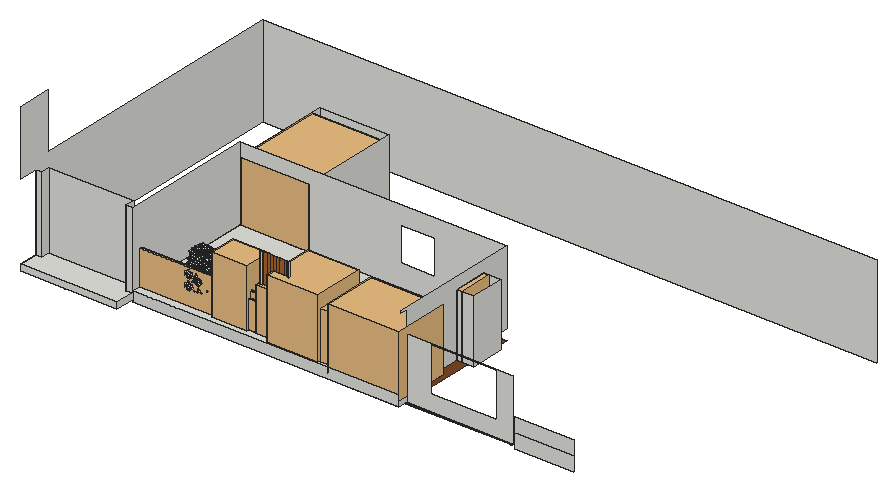
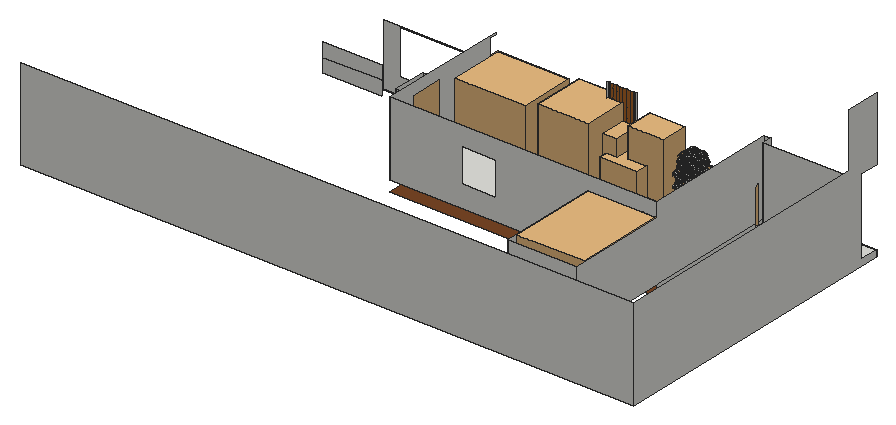
# SketchUp Ruby script. Lengths in inches.
U = 1.inch
M = Sketchup.active_model
def pt(a) = Geom::Point3d.new(a.map { |v| v * U })
def face(e, loops, mat)
  f = e.add_face(loops[0].map { |a| pt(a) })
  loops[1..].each { |l| e.add_face(l.map { |a| pt(a) }).erase! }
  f.material = f.back_material = mat if mat
  f
end
# faces: each face lists its corners as indices into pts; further lists are holes
def faces(e, pts, list, mat = nil) = list.each { |f| face(e, (f[0].is_a?(Array) ? f : [f]).map { |l| l.map { |i| pts[i] } }, mat) }
# xy, xz, yz: faces in a plane at the given z, y or x. An outline is a flat list of corners, or four numbers for a rectangle; further outlines are holes
def ring(l) = l.size == 4 ? [[l[0], l[1]], [l[2], l[1]], [l[2], l[3]], [l[0], l[3]]] : l.each_slice(2).to_a
def flat(e, list, mat, &to3) = list.each { |f| face(e, (f[0].is_a?(Array) ? f : [f]).map { |l| ring(l).map { |u, v| to3.(u, v) } }, mat) }
def xy(e, z, list, mat = nil) = flat(e, list, mat) { |x, y| [x, y, z] }
def xz(e, y, list, mat = nil) = flat(e, list, mat) { |x, z| [x, y, z] }
def yz(e, x, list, mat = nil) = flat(e, list, mat) { |y, z| [x, y, z] }
def lines(e, pts, list) = list.each { |a, b| e.add_line(pt(pts[a]), pt(pts[b])) }
# prism: a flat outline (further loops are holes) pulled along v
def prism(e, loops, v, mat = nil)
  f = face(e, loops, mat); d = Geom::Vector3d.new(v.map { |x| x * U })
  f.pushpull(f.normal.samedirection?(d) ? d.length : -d.length)
end
def box(e, o, s, mat = nil) = prism(e, [[o, [o[0] + s[0], o[1], o[2]], [o[0] + s[0], o[1] + s[1], o[2]], [o[0], o[1] + s[1], o[2]]]], [0, 0, s[2]], mat)
def at(x, y, z, deg = 0) = Geom::Transformation.translation(pt([x, y, z])) * Geom::Transformation.rotation(ORIGIN, Z_AXIS, deg.degrees)
def axes(o, x, y, z) = Geom::Transformation.new([*x, 0, *y, 0, *z, 0, *pt(o).to_a, 1])
def part(name) = M.definitions.add(name)
# library, detail: a bought-in or finely detailed component or shape, given as its bounding box
def library(name, o, s) = part(name).tap { |d| box(d.entities, o, s) }
def detail(e, o, s) = box(e.add_group.entities, o, s)
def put(e, d, t, mat = nil) = e.add_instance(d, t).tap { |i| i.material = mat if mat }
def group(e, t, mat = nil) = e.add_group.tap { |g| g.transformation = t; g.material = mat if mat }.entities
root = M.entities
M.materials.add("[Wood Bamboo]").color = [173, 103, 41]
M.materials.add("[Wood Veneer 01]").color = [120, 70, 37]
c1 = library("Tlon Light 1950 Ceiling 152 010",[-38.39,-38.39,-3.78],[76.78,76.78,3.41])
c2 = library("Rectangular Planter with Plant",[-49.93,-33.04,0],[93.24,71.01,81.08])
c3 = library("Glass Railings(black Handrails)",[-57.04,-132.55,0],[169.29,2.52,28.17])
c4 = library("Group\#14",[0,0,0],[39.5,117.4375,51.17])
c5 = library("Untitled (14)",[0,0,0],[7.13,36,83])
c6 = library("Hanging Plant\#2",[-3.24,-1.74,-0.87],[34.15,22.4,50.98])
c7 = library("Yukka Plant GHD",[0,0,0],[46.13,35.26,75.51])
c8 = library("Philodendron Plant GHD",[-18.43,-10.97,-1.09],[51.75,39.48,62.43])
c9 = library("Plant Banana",[3.49,5.74,0],[38.27,39.55,56.51])
c10 = library("Potted indoor plant",[-35.72,-28.42,0],[66.31,67.39,78.4375])
c11 = part("leaflet")
p = [[2.87,10.24,0.32],[0.33,13.79,0],[-2.24,10.39,0.32],[-2.2,6.92,0.33],[0.45,0.11,0.33],[2.91,6.86,0.33]]
faces(c11.entities,p,[[0,1,2],[0,2,3,4,5]])
c12 = part("leaf group")
put(c12.entities,c11,axes([4.25,4.04,0.04],[0.8,0,0],[0,0.8,0],[0,0,0.8]))
put(c12.entities,c11,axes([4.5,3.78,0.04],[0.4,0.69282,-0.00011],[-0.69282,0.4,-0.00008],[-0.00001,0.00014,0.8]))
put(c12.entities,c11,axes([4.92,3.9375,0.04],[-0.56569,0.56569,-0.00025],[-0.56569,-0.56569,0.00001],[-0.00017,0.00019,0.8]))
put(c12.entities,c11,axes([4.87,4.38,0.04],[-0.69282,-0.4,-0.0002],[0.4,-0.69282,0.00017],[-0.00026,0.00005,0.8]))
put(c12.entities,c11,axes([4.42,4.45,0.04],[0.20706,-0.77274,-0.00003],[0.77274,0.20706,0.00016],[-0.00015,-0.00007,0.8]))
c13 = part("branch with leaves\#1")
put(c13.entities,c12,axes([2.86,31.23,35.15],[-0.02765,-0.79009,-0.61237],[0.48114,-0.54749,0.68465],[-0.8762,-0.27571,0.39528]))
put(c13.entities,c12,axes([12.72,29.5,24.05],[-0.41566,0.90952,0],[-0.44736,-0.20444,-0.87067],[-0.7919,-0.3619,0.49186]))
put(c13.entities,c12,axes([15.91,15.09,15.29],[-0.51919,0.82474,-0.22414],[0.78767,0.35997,-0.5],[-0.33169,-0.43615,-0.83652]))
put(c13.entities,c12,axes([23.4,16.37,17.31],[0.5,0.75,-0.43301],[0,0.5,0.86603],[0.86603,-0.43301,0.25]))
put(c13.entities,c12,axes([11.3125,8.27,23.62],[1.15,0,0],[0,0.575,0.99593],[0,-0.86603,0.5]))
c14 = part("leaflet\#1")
p = [[0.33,13.79,0],[2.87,10.24,0.32],[-2.24,10.39,0.32],[2.91,6.86,0.33],[0.45,0.11,0.33],[-2.2,6.92,0.33]]
faces(c14.entities,p,[[0,1,2],[2,1,3,4,5]])
c15 = part("leaf group\#1")
put(c15.entities,c14,axes([1.8,0.82,0.04],[-0.56569,0.56569,-0.00025],[-0.33941,-0.33941,0.00001],[-0.00017,0.00019,0.8]))
c16 = part("flower")
put(c16.entities,c15,axes([3.87,3.58,0.87],[0.08758,0.98061,-0.17532],[0.93721,-0.14075,-0.31909],[-0.33758,-0.13637,-0.93137]))
put(c16.entities,c15,axes([3.58,5.87,0.87],[0.98061,-0.08758,-0.17532],[-0.14075,-0.93721,-0.31909],[-0.13637,0.33758,-0.93137]))
put(c16.entities,c15,axes([5.87,6.16,0.87],[-0.08758,-0.98061,-0.17532],[-0.93721,0.14075,-0.31909],[0.33758,0.13637,-0.93137]))
put(c16.entities,c15,axes([6.16,3.87,0.87],[-0.98061,0.08758,-0.17532],[0.14075,0.93721,-0.31909],[0.13637,-0.33758,-0.93137]))
put(c16.entities,c15,axes([4.97,4.02,1.64],[-0.54077,0.62855,-0.55902],[0.78035,0.12673,-0.61237],[-0.31406,-0.76738,-0.55902]))
put(c16.entities,c15,axes([4.08,5.2,1.64],[0.81472,0.15405,-0.55902],[-0.28042,-0.73917,-0.61237],[-0.50754,0.65567,-0.55902]))
put(c16.entities,c15,axes([5.55,5.38,1.64],[-0.27395,-0.78259,-0.55902],[-0.49993,0.61243,-0.61237],[0.8216,0.11171,-0.55902]))
c17 = part("branch")
p = [[0.27,0.14,21.6],[1.15,1.36,21.6],[2.31,4.21,0],[0.54,1.79,0],[1.05,2.55,32.4],[1.34,2.95,32.4]]
faces(c17.entities,p,[[0,1,2,3],[4,5,1,0]])
c18 = part("branch with leaves")
put(c18.entities,c12,axes([29.28,4.46,29.75],[0.70711,0.61237,-0.35355],[-0.27393,0.69819,0.66144],[0.65189,-0.37086,0.66144]))
put(c18.entities,c12,axes([2.86,31.23,35.15],[-0.02765,-0.79009,-0.61237],[0.48114,-0.54749,0.68465],[-0.8762,-0.27571,0.39528]))
put(c18.entities,c17,axes([15.22,43.9,5.2],[1,0,0],[0,0.5,0.86603],[0,-1.03923,0.6]))
put(c18.entities,c12,axes([12.72,29.5,24.05],[-0.41566,0.90952,0],[-0.44736,-0.20444,-0.87067],[-0.7919,-0.3619,0.49186]))
put(c18.entities,c12,axes([15.91,15.09,15.29],[-0.51919,0.82474,-0.22414],[0.78767,0.35997,-0.5],[-0.33169,-0.43615,-0.83652]))
put(c18.entities,c12,axes([31.61,42.03,14.23],[-0.02765,-0.79009,-0.61237],[0.47126,0.52995,-0.70503],[0.88156,-0.30808,0.35768]))
put(c18.entities,c12,axes([23.4,16.37,17.31],[0.5,0.75,-0.43301],[0,0.5,0.86603],[0.86603,-0.43301,0.25]))
put(c18.entities,c12,axes([12.04,8.6,24.1875],[1,0,0],[0,0.5,0.86603],[0,-0.86603,0.5]))
c19 = part("trunk")
p = [[2.07,0,0],[2.91,2.57,208.4],[2.76,2.68,208.4],[0.57,1.09,0],[3.93,0,0],[3.09,2.57,208.4],
  [5.43,1.09,0],[3.24,2.68,208.4],[2.7,2.85,208.4],[0,2.85,0],[6,2.85,0],[3.3,2.85,208.4],
  [2.76,3.03,208.4],[0.57,4.62,0],[5.43,4.62,0],[3.24,3.03,208.4],[2.91,3.14,208.4],[2.07,5.71,0],
  [3.93,5.71,0],[3.09,3.14,208.4]]
faces(c19.entities,p,[[0,1,2,3],[4,5,1,0],[6,7,5,4],[3,2,8,9],[6,10,11,7],[8,12,13,9],[11,10,14,15],[13,12,16,17],
  [18,19,15,14],[17,16,19,18]])
c20 = part("Flowering tree")
put(c20.entities,c13,axes([8.5625,69.79,58.85],[-1.14545,-0.10223,0],[0.09875,-1.10642,-0.25882],[0.02646,-0.29646,0.96593]))
put(c20.entities,c16,axes([18.03,-59.9,126.47],[-1.06473,0.02061,0.37747],[-0.32263,-0.80708,-0.6548],[0.29115,-0.81896,0.6548]))
put(c20.entities,c16,axes([24.99,-51.52,163.52],[0.99593,0.2875,-0.43301],[0,0.99593,0.5],[0.575,-0.49796,0.75]))
put(c20.entities,c16,axes([9.15,43.86,180.9375],[-0.776,0.32151,0.68301],[0.59221,-0.55726,0.70711],[0.60796,0.9532,0.18301]))
put(c20.entities,c16,axes([-19.44,51.82,88.4375],[-0.978,0.2192,-0.49033],[-0.25151,-1.12216,0],[-0.55023,0.12332,0.87153]))
put(c20.entities,c13,axes([79.24,-48.01,132.64],[0.21275,1.12031,-0.12941],[-1.10684,0.17595,-0.22414],[-0.22834,0.19092,0.96593]))
put(c20.entities,c13,axes([64.36,-6.43,165.85],[-0.10223,1.14545,0],[-1.10642,-0.09875,-0.25882],[-0.29646,-0.02646,0.96593]))
put(c20.entities,c13,axes([52.57,39.62,163.85],[-0.88224,0.73767,0],[-0.71253,-0.85218,-0.25882],[-0.19092,-0.22834,0.96593]))
put(c20.entities,c13,axes([-64.4,-29.26,175.85],[0.88224,-0.73767,0],[0.71253,0.85218,-0.25882],[0.19092,0.22834,0.96593]))
put(c20.entities,c13,axes([40.35,-16.55,200.81],[-0.14358,1.14093,0.01256],[-0.77283,-0.08933,-0.72016],[-0.83795,-0.11311,0.69546]))
put(c20.entities,c13,axes([7.875,84.56,112.85],[-1.14773,-0.07221,0],[0.06975,-1.10862,-0.25882],[0.01869,-0.29705,0.96593]))
put(c20.entities,c13,axes([-66.42,6.43,163.85],[0.10223,-1.14545,0],[1.10642,0.09875,-0.25882],[0.29646,0.02646,0.96593]))
put(c20.entities,c13,axes([-6.02,-66.82,162.85],[1.14545,0.10223,0],[-0.09875,1.10642,-0.25882],[-0.02646,0.29646,0.96593]))
put(c20.entities,c13,axes([65.22,55.72,70.85],[-0.88224,0.73767,0],[-0.71253,-0.85218,-0.25882],[-0.19092,-0.22834,0.96593]))
put(c20.entities,c13,axes([-6.02,-85.22,100.85],[1.14545,0.10223,0],[-0.09875,1.10642,-0.25882],[-0.02646,0.29646,0.96593]))
put(c20.entities,c13,axes([-64.4,-55.71,70.85],[0.88224,-0.73767,0],[0.71253,0.85218,-0.25882],[0.19092,0.22834,0.96593]))
put(c20.entities,c13,axes([-46.27,-12.7,180.74],[-0.29529,-0.0373,-0.96593],[1.10206,0.13922,-0.25882],[0.14413,-1.14093,0]))
put(c20.entities,c13,axes([56.125,-64.81,70.85],[0.73767,0.88224,0],[-0.85218,0.71253,-0.25882],[-0.22834,0.19092,0.96593]))
put(c20.entities,c13,axes([-55.31,64.8125,78.85],[-0.73767,-0.88224,0],[0.85218,-0.71253,-0.25882],[0.22834,-0.19092,0.96593]))
put(c20.entities,c13,axes([-84.82,6.43,92.85],[0.10223,-1.14545,0],[1.10642,0.09875,-0.25882],[0.29646,0.02646,0.96593]))
put(c20.entities,c18,axes([56.87,3.27,57.34],[-0.44564,1.06014,0],[-1.06014,-0.44564,0],[0,0,1]))
put(c20.entities,c16,axes([-46.02,24.68,176.39],[-0.60389,-0.88348,0.36612],[0.59197,0.06424,0.85552],[-0.77935,0.73337,0.36612]))
put(c20.entities,c18,axes([-18.99,-54,51.28],[1.15,0,0],[0,1.15,0],[0,0,1]))
put(c20.entities,c16,axes([-14.26,69.05,133.89],[-0.21654,-1.04563,0.37124],[1.09634,-0.09014,0.29155],[-0.27139,0.47014,0.88158]))
put(c20.entities,c13,axes([7.875,59.26,173.85],[-1.14773,-0.07221,0],[0.06975,-1.10862,-0.25882],[0.01869,-0.29705,0.96593]))
put(c20.entities,c16,axes([-39.65,-46.59,156.55],[0.81317,-0.40659,0.61237],[0,0.99593,0.5],[-0.81317,-0.40659,0.61237]))
put(c20.entities,c13,axes([68.45,-14.73,133.12],[0.31285,1.10009,0.10445],[-1.0665,0.33304,-0.23681],[-0.29529,-0.0373,0.96593]))
put(c20.entities,c18,axes([-54.71,-13.99,125.23],[0.64805,-0.95001,0],[0.91764,0.62597,-0.25882],[0.24588,0.16773,0.96593]))
put(c20.entities,c16,axes([-59.37,-17.76,103.29],[0.82621,-0.65851,-0.39489],[0.59197,0.06424,0.85552],[-0.538,-0.9406,0.33489]))
put(c20.entities,c18,axes([-55.12,-14.55,89.35],[0.64805,-0.95001,0],[0.91764,0.62597,-0.25882],[0.24588,0.16773,0.96593]))
put(c20.entities,c16,axes([48.53,-28.74,71.58],[0.35234,0.10813,0.94725],[-0.36862,-1.06582,0.19567],[1.03076,-0.41812,-0.25382]))
put(c20.entities,c13,axes([-12.83,63.67,197.61],[0.0612,-1.14229,0.10265],[-1.10726,-0.09004,-0.2585],[0.30453,-0.09784,-0.96054]))
put(c20.entities,c13,axes([-64.4,-55.71,112.85],[0.88224,-0.73767,0],[0.71253,0.85218,-0.25882],[0.19092,0.22834,0.96593]))
put(c20.entities,c13,axes([65.22,55.72,114.85],[-0.88224,0.73767,0],[-0.71253,-0.85218,-0.25882],[-0.19092,-0.22834,0.96593]))
put(c20.entities,c16,axes([63.34,2.95,120.74],[0.8666,0.37799,-0.5693],[-0.45977,1.05409,0],[0.6001,0.26175,0.82213]))
put(c20.entities,c13,axes([85.63,-6.43,94.85],[-0.10223,1.14545,0],[-1.10642,-0.09875,-0.25882],[-0.29646,-0.02646,0.96593]))
put(c20.entities,c18,axes([31.42,47.13,103.94],[-1.11535,0.28016,0],[-0.27473,-1.09373,-0.19595],[-0.0549,-0.21855,0.98061]))
put(c20.entities,c19,axes([-3.39,-3.28,43.76],[1.15,0,0],[0,1.15,0],[0,0,0.79]))
put(c20.entities,c18,axes([34.9,-44.92,95.18],[0.62465,0.96556,0],[-0.93266,0.60337,-0.25882],[-0.24991,0.16167,0.96593]))
put(c20.entities,c18,axes([32.7,-43.8,134.99],[0.62465,0.96556,0],[-0.88615,0.57328,-0.39715],[-0.38347,0.24808,0.91775]))
put(c20.entities,c13,axes([-51.54,49.67,143.57],[0.26379,-0.52212,-0.86096],[0.65423,-0.75347,0.49708],[-0.90824,-0.69439,0.108]))
put(c20.entities,c18,axes([31.48,46.68,140.85],[-1.11535,0.28016,0],[-0.27061,-1.07735,-0.25882],[-0.07251,-0.28867,0.96593]))
put(c20.entities,c13,axes([8.75,19.55,179.21],[-0.27543,0.79346,0.68307],[-1.10726,-0.09004,-0.2585],[-0.14361,-0.82754,0.68307]))
c21 = part("Plant GHD")
put(c21.entities,c20,axes([21.36,20.42,-5.32],[0.2847,0,0],[0,0.2847,0],[0,0,0.33025]))
g1 = group(c21.entities,at(14.85,13.9,0))
detail(g1,[0,0,0],[13.04,13.04,11.8])
c22 = library("Group\#719",[-5.55,-6.67,0],[49.65,49.64,35.75])
c23 = part("Plants indoor GHD")
put(c23.entities,c6,at(254.34,21.02,0))
put(c23.entities,c7,at(45.23,2.59,0))
put(c23.entities,c8,at(201.7,11.53,0))
put(c23.entities,c9,at(99.46,-3.08,1.17))
put(c23.entities,c10,at(158.24,24.68,0))
put(c23.entities,c21,at(0,0,0))
put(c23.entities,c22,at(72.51,10.66,1.17))
xy(root,360.26,[[563.03,893.4375,564.64,916.1875]])
xy(root,360.64,[[973.0625,915.15,1112.75,916.1875]])
xy(root,361.64,[[973.0625,915.15,1112.75,916.1875]])
xy(root,361.64,[[624.25,904.1875,973.0625,1080.1875]],"[Wood Veneer 01]")
xy(root,364.51,[[497.625,879.3125,497.625,904.1875,510,904.1875,510,916.1875,616.25,916.1875,616.25,904.1875,624.25,904.1875,624.25,879.3125],[497.625,904.1875,510,916.1875],[616.25,904.1875,624.25,916.1875]])
xy(root,372.51,[[497.625,879.3125,624.25,879.3125,624.25,904.1875,616.25,904.1875,616.25,916.1875,505.625,916.1875,505.625,904.1875,497.625,904.1875],[497.625,904.1875,505.625,916.1875],[616.25,904.1875,624.25,916.1875]])
xy(root,375.26,[[624.25,904.1875,973.0625,904.1875,973.0625,998.1875,995.625,998.1875,995.625,1042.875,973.0625,1042.875,973.0625,1080.1875,714.02,1080.1875,714.02,1211.5,624.25,1211.5],[782.66,915.1875,785.84,916.1875],[817.03,915.1875,820.03,916.1875]])
xz(root,879.3125,[[497.625,364.51,624.25,372.51]])
xz(root,904.1875,[[624.25,361.64,973.0625,375.26],[497.625,372.51,505.625,472.51],[616.25,372.51,624.25,472.51]])
xz(root,915.15,[[973.0625,360.64,1112.75,361.64]])
xz(root,915.1875,[[782.66,375.26,785.84,472.51],[817.03,375.26,820.03,472.51]])
xz(root,916.1875,[[[973.0625,361.64,1112.75,441.7],[1005.21,382.92,1091.46,440.98]],[505.625,372.51,616.25,472.51]])
xz(root,916.1875,[[785.84,375.26,790.3,472.51],[790.3,375.26,794.75,472.51],[794.75,375.26,799.21,472.51],[799.21,375.26,803.67,472.51],[803.67,375.26,808.12,472.51],
  [808.12,375.26,812.58,472.51],[812.58,375.26,817.03,472.51]],"[Wood Bamboo]")
xz(root,919.75,[[1112.75,354.31,1189.1875,372.91],[1112.75,372.91,1189.1875,391.51]])
xz(root,998.1875,[[973.0625,375.26,995.625,457.58]])
xz(root,1042.875,[[973.0625,375.26,995.625,457.58]])
xz(root,1080.1875,[[[714.02,375.26,973.0625,375.26,973.0625,472.51,624.25,472.51,624.25,454.24,714.02,454.24],[834.07,403.73,878.82,448.48]]])
xz(root,1211.5,[[624.25,375.26,714.02,454.24]])
xz(root,1276.1875,[[497.625,364.51,1299.8125,484.51]])
yz(root,497.625,[[879.3125,364.51,879.3125,372.51,904.1875,372.51,904.1875,472.51,879.3125,472.51,879.3125,556.51,924.1875,556.51,924.1875,484.51,1276.1875,484.51,1276.1875,364.51]])
yz(root,505.625,[[904.1875,372.51,916.1875,472.51]])
yz(root,616.25,[[904.1875,372.51,916.1875,472.51]])
yz(root,624.25,[[904.1875,361.64,916.1875,364.51],[916.1875,361.64,1080.1875,361.64,1080.1875,375.26,904.1875,375.26,904.1875,364.51,916.1875,364.51],[879.3125,364.51,904.1875,372.51],[904.1875,375.26,1211.5,375.26,1211.5,454.24,1080.1875,454.24,1080.1875,472.51,904.1875,472.51]])
yz(root,714.02,[[1080.1875,375.26,1211.5,454.24]])
yz(root,782.66,[[915.1875,375.26,916.1875,472.51]])
yz(root,785.84,[[915.1875,375.26,916.1875,472.51]],"[Wood Bamboo]")
yz(root,817.03,[[915.1875,375.26,916.1875,472.51]],"[Wood Bamboo]")
yz(root,820.03,[[915.1875,375.26,916.1875,472.51]])
yz(root,973.0625,[[904.1875,361.64,916.1875,375.26],[916.1875,375.26,916.1875,441.7,907.15,441.7,907.15,444.51,916.1875,444.51,916.1875,469.7,907.15,469.7,907.15,472.51,1080.1875,472.51,1080.1875,375.26,1042.875,375.26,1042.875,457.58,998.1875,457.58,998.1875,375.26]])
yz(root,995.625,[[998.1875,375.26,1042.875,457.58]])
p = [[546.34,916.1875,354.875],[545.04,916.1875,353.93],[545.04,893.4375,353.93],[546.34,893.4375,354.875],[582.61,916.1875,353.86],[581.31,916.1875,354.8125],
  [581.31,893.4375,354.8125],[582.61,893.4375,353.86],[579.96,916.1875,355.7],[579.96,893.4375,355.7],[547.7,916.1875,355.75],[547.7,893.4375,355.75],
  [578.56,916.1875,356.51],[578.56,893.4375,356.51],[549.1,916.1875,356.56],[549.1,893.4375,356.56],[577.12,916.1875,357.24],[577.12,893.4375,357.24],
  [550.54,916.1875,357.29],[550.54,893.4375,357.29],[575.64,916.1875,357.9],[575.64,893.4375,357.9],[552.02,916.1875,357.94],[552.02,893.4375,357.94],
  [553.53,916.1875,358.52],[553.53,893.4375,358.52],[574.14,916.1875,358.48],[574.14,893.4375,358.48],[555.07,916.1875,359.02],[555.07,893.4375,359.02],
  [572.6,916.1875,358.99],[572.6,893.4375,358.99],[556.63,916.1875,359.43],[556.63,893.4375,359.43],[571.04,916.1875,359.41],[571.04,893.4375,359.41],
  [558.21,916.1875,359.77],[558.21,893.4375,359.77],[569.46,916.1875,359.75],[569.46,893.4375,359.75],[567.86,916.1875,360],[567.86,893.4375,360],
  [559.81,916.1875,360.02],[559.81,893.4375,360.02],[561.41,916.1875,360.18],[561.41,893.4375,360.18],[566.26,916.1875,360.17],[566.26,893.4375,360.17],
  [563.03,916.1875,360.26],[563.03,893.4375,360.26],[564.64,916.1875,360.26],[564.64,893.4375,360.26],[624.25,916.1875,375.58],[624.25,916.1875,375.26],
  [973.0625,1080.1875,361.64],[973.0625,1080.1875,375.26]]
faces(root,p,[[0,1,2,3],[4,5,6,7],[5,8,9,6],[10,0,3,11],[8,12,13,9],[14,10,11,15],[12,16,17,13],[18,14,15,19],
  [16,20,21,17],[22,18,19,23],[24,22,23,25],[20,26,27,21],[28,24,25,29],[26,30,31,27],[32,28,29,33],[30,34,35,31],
  [36,32,33,37],[34,38,39,35],[38,40,41,39],[42,36,37,43],[44,42,43,45],[40,46,47,41],[48,44,45,49],[46,50,51,47]])
lines(root,p,[[52,53],[54,55]])
put(root,c1,axes([890.24,983.24,361.7],[0.16,0,0],[0,0.16,0],[0,0,0.16]))
put(root,c1,axes([696.92,983.24,361.7],[0.16,0,0],[0,0.16,0],[0,0,0.16]))
put(root,c2,at(929.76,937.23,368.18))
put(root,c3,axes([677.61,1047.74,372.65],[0.9357,0,0],[0,1,0],[0,0,1.70393]))
put(root,c3,axes([871.44,1047.92,374.75],[0.90532,0,0],[0,1,0],[0,0,1.70393]))
put(root,c4,axes([624.75,1080.1875,375.26],[2.26,0,0],[0,1,0],[0,0,1.54351]))
put(root,c5,axes([973.0625,998.1875,375.26],[1,0,0],[0,1.24132,0],[0,0,0.99172]))
put(root,c23,at(677.54,907.93,376.36))
